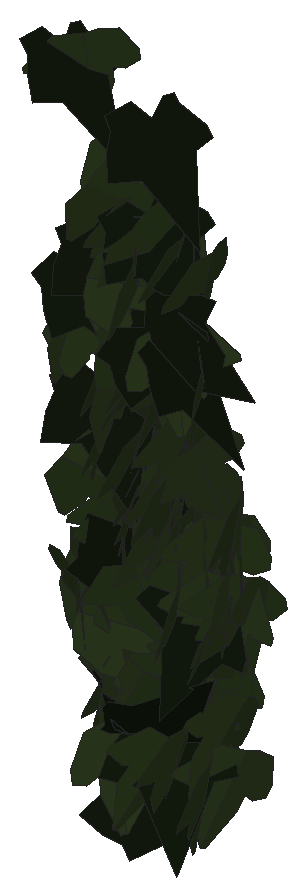
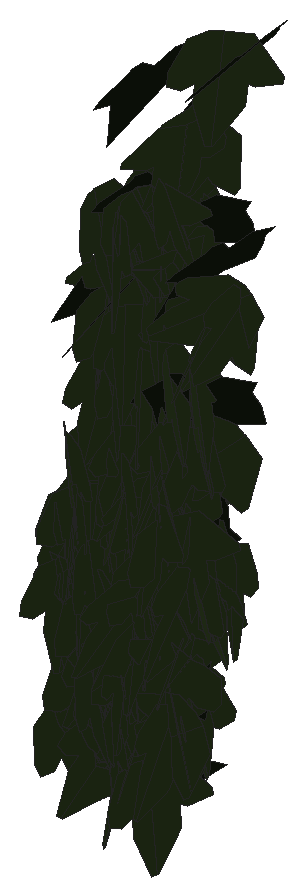
# SketchUp Ruby script. Lengths in inches.
U = 1.inch
M = Sketchup.active_model
def pt(a) = Geom::Point3d.new(a.map { |v| v * U })
def face(e, loops, mat)
  f = e.add_face(loops[0].map { |a| pt(a) })
  loops[1..].each { |l| e.add_face(l.map { |a| pt(a) }).erase! }
  f.material = f.back_material = mat if mat
  f
end
# faces: each face lists its corners as indices into pts; further lists are holes
def faces(e, pts, list, mat = nil) = list.each { |f| face(e, (f[0].is_a?(Array) ? f : [f]).map { |l| l.map { |i| pts[i] } }, mat) }
# xy, xz, yz: faces in a plane at the given z, y or x. An outline is a flat list of corners, or four numbers for a rectangle; further outlines are holes
def ring(l) = l.size == 4 ? [[l[0], l[1]], [l[2], l[1]], [l[2], l[3]], [l[0], l[3]]] : l.each_slice(2).to_a
def flat(e, list, mat, &to3) = list.each { |f| face(e, (f[0].is_a?(Array) ? f : [f]).map { |l| ring(l).map { |u, v| to3.(u, v) } }, mat) }
def xy(e, z, list, mat = nil) = flat(e, list, mat) { |x, y| [x, y, z] }
def xz(e, y, list, mat = nil) = flat(e, list, mat) { |x, z| [x, y, z] }
def yz(e, x, list, mat = nil) = flat(e, list, mat) { |y, z| [x, y, z] }
def lines(e, pts, list) = list.each { |a, b| e.add_line(pt(pts[a]), pt(pts[b])) }
# prism: a flat outline (further loops are holes) pulled along v
def prism(e, loops, v, mat = nil)
  f = face(e, loops, mat); d = Geom::Vector3d.new(v.map { |x| x * U })
  f.pushpull(f.normal.samedirection?(d) ? d.length : -d.length)
end
def box(e, o, s, mat = nil) = prism(e, [[o, [o[0] + s[0], o[1], o[2]], [o[0] + s[0], o[1] + s[1], o[2]], [o[0], o[1] + s[1], o[2]]]], [0, 0, s[2]], mat)
def at(x, y, z, deg = 0) = Geom::Transformation.translation(pt([x, y, z])) * Geom::Transformation.rotation(ORIGIN, Z_AXIS, deg.degrees)
def axes(o, x, y, z) = Geom::Transformation.new([*x, 0, *y, 0, *z, 0, *pt(o).to_a, 1])
def part(name) = M.definitions.add(name)
# library, detail: a bought-in or finely detailed component or shape, given as its bounding box
def library(name, o, s) = part(name).tap { |d| box(d.entities, o, s) }
def detail(e, o, s) = box(e.add_group.entities, o, s)
def put(e, d, t, mat = nil) = e.add_instance(d, t).tap { |i| i.material = mat if mat }
def group(e, t, mat = nil) = e.add_group.tap { |g| g.transformation = t; g.material = mat if mat }.entities
root = M.entities
M.materials.add("efeu1").color = [18, 25, 13]
M.materials.add("efeu2").color = [43, 57, 29]
c1 = part("ivyleaf_10")
p = [[0,0.5,-0.03],[-0.0625,2.02,-0.43],[-0.19,2.01,-0.46],[-0.54,1.05,-0.29],[-0.52,0.625,-0.18],[-0.83,0.76,-0.28],
  [-1.16,0.64,-0.33],[-1.15,0.33,-0.24],[-0.77,-0.39,0.02],[-0.3,-0.51,0.16],[0.04,-0.48,0.23],[-0.02,2.01,-0.4375],
  [-0.06,2.01,-0.43],[0.04,-0.49,0.23],[0.67,-0.49,0.14],[1.38,0.36,-0.2],[1.375,0.51,-0.24],[0.81,0.65,-0.19],
  [0.62,0.59,-0.15],[0.6,1.09,-0.28],[0.5,1.23,-0.31]]
faces(c1.entities,p,[[0,1,2,3,4,5,6,7,8,9,10],[11,12,0,13,14,15,16,17,18,19,20]],"efeu2")
c2 = part("ivyleaf_9")
p = [[1.54,2.16,1.25],[1.36,2.04,1.19],[-0.21,0.99,0.68],[-0.71,1.11,0.82],[-0.85,0.86,0.67],[-0.8,0.17,0.21],
  [-0.9,-0.01,0.1],[-0.67,-0.16,-0.02],[-0.08,-0.08,-0.05],[-0.03,-0.6,-0.4],[0.65,-0.88,-0.66],[0.83,-0.6,-0.49],
  [1.29,-0.42,-0.43],[1.8125,-0.07,-0.26],[1.21,0.44,0.15]]
faces(c2.entities,p,[[0,1,2,3,4,5,6,7,8,9,10,11,12,13,14]],"efeu1")
put(root,c1,axes([15.91,224.3125,216.32],[0.3264,-0.17803,-0.33432],[-0.1434,0.35039,-0.3266],[0.35057,0.30908,0.17768]))
put(root,c1,axes([15.86,224.61,222.82],[-0.35248,-0.35123,-0.049],[0.0485,0.0207,-0.49721],[0.3513,-0.35526,0.01948]))
put(root,c1,axes([15.82,224.41,219.51],[-0.03059,-0.26658,-0.4219],[0.11756,0.40695,-0.26566],[0.48502,-0.11546,0.03778]))
put(root,c1,axes([15.85,225.21,216.42],[-0.05418,-0.35899,-0.34378],[0.08898,0.33323,-0.36199],[0.48903,-0.10041,0.02778]))
put(root,c1,axes([15.89,225.47,214.83],[-0.06009,-0.37722,-0.32264],[0.05139,0.31852,-0.38197],[0.49371,-0.07906,0.00049]))
put(root,c1,axes([15.93,224.9,218.89],[0.17932,-0.454,-0.10828],[-0.01653,0.10974,-0.48753],[0.46644,0.17843,0.02435]))
put(root,c1,axes([15.91,224.83,216.34],[0.21325,-0.44852,0.05793],[0.02073,-0.05429,-0.49661],[0.45177,0.21421,-0.00455]))
put(root,c2,axes([15.6875,224.48,222.81],[0.19731,-0.4431,-0.12137],[0.03083,0.14457,-0.47765],[0.45839,0.18101,0.08437]))
put(root,c1,axes([16.04,225.2,217.02],[-0.27324,-0.41488,0.0567],[-0.01893,-0.0554,-0.49656],[0.41831,-0.2735,0.01457]))
put(root,c1,axes([16.02,224.92,215.07],[0.14589,-0.47813,-0.01052],[0.00012,0.01104,-0.49988],[0.47824,0.14585,0.00334]))
put(root,c1,axes([15.67,224.65,216.34],[0.10547,-0.02634,0.48804],[0.46803,-0.13839,-0.10861],[0.1408,0.47975,-0.00454]))
put(root,c1,axes([15.74,225.4375,214.87],[-0.29243,0.07265,-0.39901],[0.39338,-0.06887,-0.30084],[-0.09867,-0.48988,-0.01688]))
put(root,c1,axes([16.08,225.11,215.03],[0.2408,-0.4293,-0.08783],[-0.033,0.08217,-0.4921],[0.43695,0.24279,0.01124]))
put(root,c1,axes([15.77,225.39,215.61],[0.37606,0.18322,0.27387],[0.25184,0.10818,-0.41818],[-0.2125,0.45247,-0.01092]))
put(root,c1,axes([16.12,225.5,214.13],[-0.20782,-0.45476,-0.00225],[-0.00216,0.00346,-0.49998],[0.45476,-0.20781,-0.0034]))
put(root,c1,axes([15.95,225.38,215.27],[-0.15026,0.18638,0.43896],[0.23977,-0.3683,0.23846],[0.41222,0.28217,0.02131]))
put(root,c1,axes([16.06,225.09,216.44],[-0.45157,-0.11332,-0.18233],[0.18209,0.02273,-0.46511],[0.1137,-0.48646,0.02075]))
put(root,c1,axes([16.15,224.84,217.03],[0.0182,-0.45408,0.20852],[0.06908,-0.20437,-0.45107],[0.49487,0.04522,0.0553]))
put(root,c1,axes([16.2,224.57,218.37],[0.19363,-0.45223,-0.0894],[-0.02976,0.0845,-0.49191],[0.46003,0.19581,0.00581]))
put(root,c1,axes([15.98,224.4,217.82],[-0.2535,-0.15705,-0.40134],[0.34718,0.20147,-0.29812],[0.25535,-0.42982,0.00691]))
put(root,c1,axes([16.24,224.96,218.91],[0.16756,-0.46558,-0.07184],[-0.00818,0.07336,-0.49452],[0.47102,0.1669,0.01696]))
put(root,c2,axes([15.98,224.38,220.26],[0.17839,-0.38394,-0.26602],[0.00861,0.28742,-0.40904],[0.46702,0.14135,0.10916]))
put(root,c1,axes([15.93,224.4,219.62],[-0.15181,-0.18195,-0.44028],[0.42072,0.16558,-0.21349],[0.22349,-0.43529,0.10283]))
put(root,c1,axes([16.24,224.8,216.94],[0.27614,-0.32312,-0.26332],[-0.00852,0.31143,-0.39108],[0.41674,0.22047,0.16649]))
put(root,c1,axes([16.31,225.34,216.55],[-0.18362,-0.46266,0.04723],[-0.01216,-0.04599,-0.49773],[0.4649,-0.18393,0.00563]))
put(root,c1,axes([16.21,224.89,217.96],[-0.18813,-0.38015,-0.26476],[0.11941,0.23631,-0.42415],[0.44761,-0.22281,0.00187]))
put(root,c2,axes([16.09,224.7,218.64],[-0.1689,-0.36114,-0.30175],[0.14601,0.26456,-0.39836],[0.44739,-0.22268,0.01609]))
put(root,c1,axes([16.36,225.32,217.17],[-0.48678,0.07054,0.08983],[-0.09096,-0.00162,-0.49165],[-0.06907,-0.495,0.01441]))
put(root,c1,axes([16.32,224.32,218.91],[0.11409,-0.22495,-0.43172],[0.03363,0.446,-0.2235],[0.48565,0.02196,0.1169]))
put(root,c1,axes([16.4,224.95,217.7],[0.13089,-0.45332,-0.16544],[-0.04834,0.15824,-0.47183],[0.48014,0.13951,-0.0024]))
put(root,c1,axes([16.59,224.62,215.22],[-0.40654,-0.14734,0.25103],[-0.23719,-0.08225,-0.43241],[0.16872,-0.47066,-0.00301]))
put(root,c1,axes([16.47,225.38,215.93],[-0.4607,0.1672,0.09902],[-0.1016,0.00993,-0.48947],[-0.16564,-0.47111,0.02483]))
put(root,c1,axes([16.3,224.71,221.67],[0.20462,0.45615,0.00785],[0.00074,0.00827,-0.49993],[-0.45621,0.2046,0.00271]))
put(root,c1,axes([16.45,225.3125,215.41],[-0.23825,-0.43837,-0.03268],[0.01271,0.03028,-0.49892],[0.4394,-0.23857,-0.00328]))
put(root,c1,axes([16.41,224.8,217.43],[0.23906,-0.439,-0.01132],[-0.00094,0.01238,-0.49985],[0.43915,0.23901,0.0051]))
put(root,c2,axes([16.125,224.86,214.85],[0.34799,-0.35875,0.01413],[0.00766,-0.01226,-0.49979],[0.35895,0.34806,-0.00303]))
put(root,c1,axes([16.4375,224.68,220.97],[0.02425,-0.49125,0.08991],[0.02321,-0.08881,-0.4915],[0.49887,0.02802,0.0185]))
put(root,c1,axes([16.37,224.73,215.57],[-0.03972,-0.34886,-0.35597],[0.12483,0.33876,-0.34592],[0.48253,-0.11635,0.06019]))
put(root,c1,axes([16.46,224.68,218.08],[0.11779,-0.48213,-0.0606],[-0.01222,0.05939,-0.49631],[0.48577,0.1184,0.00221]))
put(root,c1,axes([16.41,225.1,217.53],[-0.2551,0.42938,-0.02363],[0.01258,-0.02001,-0.49944],[-0.42985,-0.25541,-0.0006]))
put(root,c1,axes([16.52,225.25,214.79],[-0.16692,-0.3801,0.27867],[-0.00651,-0.29374,-0.40456],[0.47127,-0.13869,0.09311]))
put(root,c1,axes([16.4,225.51,215.86],[-0.06336,0.47744,-0.1343],[0.00339,-0.13497,-0.48143],[-0.49596,-0.06191,0.01386]))
put(root,c1,axes([16.32,225.57,216.3125],[-0.13509,-0.3874,-0.28578],[0.26213,0.18977,-0.38115],[0.40378,-0.2528,0.15183]))
put(root,c1,axes([16.49,225.38,215.46],[-0.00687,-0.46531,-0.18287],[0.04683,0.18148,-0.46354],[0.49775,-0.0235,0.04109]))
put(root,c1,axes([16.39,224.21,221.44],[-0.20414,-0.27553,-0.36388],[0.19752,0.30603,-0.34254],[0.41148,-0.2836,-0.0161]))
put(root,c1,axes([16.11,225.3,216.16],[0.21621,0.02595,0.45009],[0.43806,0.10591,-0.21653],[-0.10658,0.48796,0.02306]))
put(root,c1,axes([16.53,225.21,216.18],[0.32149,-0.34519,-0.16578],[-0.04518,0.18076,-0.46399],[0.38027,0.31332,0.08503]))
put(root,c1,axes([16.42,224.32,219.85],[0.0741,0.15398,-0.46989],[0.16765,0.43918,0.17035],[0.46519,-0.1828,0.01346]))
put(root,c1,axes([16.28,224.35,216.01],[0.10152,0.12077,0.47446],[0.23427,0.41349,-0.15537],[-0.4299,0.25385,0.02737]))
put(root,c1,axes([16.8,224.47,217.46],[0.20163,-0.07105,0.45199],[-0.42082,0.16508,0.21367],[-0.17959,-0.46658,0.00677]))
put(root,c2,axes([16.35,224.49,220.7],[-0.12105,-0.3658,-0.31864],[0.13884,0.28856,-0.38401],[0.46483,-0.18145,0.03171]))
put(root,c2,axes([16.75,224.8125,213.61],[-0.34451,-0.35475,0.0739],[0.05805,0.04662,0.49443],[-0.35769,0.34925,0.00907]))
put(root,c1,axes([16.61,225.125,214.96],[-0.10935,-0.35626,0.33335],[-0.00065,-0.34152,-0.36519],[0.4879,-0.0803,0.07423]))
put(root,c1,axes([16.45,224.46,214.51],[0.30504,0.39535,0.02547],[0.01524,0.02041,-0.49935],[-0.39588,0.30542,0.00041]))
put(root,c1,axes([16.61,224.98,218.79],[0.13265,-0.40051,-0.26832],[-0.03725,0.26894,-0.41986],[0.48064,0.13138,0.04152]))
put(root,c1,axes([16.67,224.93,220.76],[-0.38481,-0.26177,0.18274],[-0.05538,-0.22714,-0.44198],[0.31441,-0.36039,0.14582]))
put(root,c1,axes([16.65,224.79,220.77],[-0.17812,-0.46386,0.05577],[-0.01443,-0.0542,-0.49684],[0.46698,-0.1786,0.00592]))
put(root,c1,axes([16.58,225.37,214.125],[-0.30917,0.39257,0.01735],[-0.00939,0.01469,-0.4997],[-0.39285,-0.30931,-0.00171]))
put(root,c2,axes([16.45,224.54,216.49],[-0.16588,-0.0569,0.46824],[0.46938,0.02905,0.16982],[-0.04654,0.4959,0.04378]))
put(root,c1,axes([16.76,224.28,220.48],[0.1054,-0.39367,-0.28968],[-0.01924,0.29277,-0.40486],[0.48839,0.09649,0.04657]))
put(root,c1,axes([17,225.4,215.61],[-0.37027,-0.06527,0.3296],[-0.32435,-0.05864,-0.37598],[0.08774,-0.49224,0.00108]))
put(root,c1,axes([16.77,225.11,217.52],[0.29694,-0.35439,-0.19036],[-0.05016,0.20213,-0.45456],[0.39914,0.28905,0.08449]))
put(root,c1,axes([16.44,225.23,214.53],[0.24527,0.20109,0.38653],[0.28437,0.26219,-0.31685],[-0.33012,0.37526,0.01424]))
put(root,c1,axes([16.73,225.43,214.63],[0.36063,-0.33396,-0.09171],[0.00485,0.13727,-0.48076],[0.34629,0.34587,0.10225]))
put(root,c1,axes([16.7,224.79,217.22],[0.00028,0.49208,0.08862],[-0.01815,0.08858,-0.49176],[-0.49967,-0.00294,0.01791]))
put(root,c1,axes([16.75,224.44,216.67],[-0.39705,-0.27846,-0.1217],[0.09958,0.06995,-0.48496],[0.28711,-0.40935,-0.00009]))
put(root,c1,axes([16.63,224.0625,220.43],[0.05117,0.16237,0.47013],[0.07833,0.46408,-0.1688],[-0.49117,0.09092,0.02206]))
put(root,c1,axes([16.83,224.48,219.39],[0.0879,-0.46509,-0.16113],[-0.0233,0.15957,-0.47328],[0.49166,0.09072,0.00638]))
put(root,c1,axes([16.86,224.7,214.47],[-0.07029,-0.39987,0.29183],[-0.02248,-0.29187,-0.40534],[0.49452,-0.07011,0.02306]))
put(root,c1,axes([16.78,224.93,217.73],[-0.16465,-0.37851,-0.28217],[0.11084,0.25949,-0.41277],[0.45892,-0.19848,-0.00154]))
put(root,c1,axes([16.79,224.38,220.9],[-0.14085,-0.39968,-0.26536],[0.10679,0.24351,-0.42344],[0.46771,-0.17596,0.01677]))
put(root,c1,axes([16.875,225.5,215.16],[0.04651,-0.49767,0.01262],[0.00087,-0.01259,-0.49984],[0.49783,0.04652,-0.0003]))
put(root,c1,axes([16.86,225.15,220.47],[0.32952,-0.31532,-0.20491],[-0.02947,0.24996,-0.43203],[0.37489,0.29681,0.14615]))
put(root,c1,axes([17.04,224.88,218.68],[-0.15225,0.30068,0.36934],[-0.30482,0.23641,-0.31811],[-0.36593,-0.32203,0.11132]))
put(root,c1,axes([16.89,224.59,217.16],[-0.0747,-0.46305,-0.17323],[0.03876,0.16917,-0.46891],[0.49287,-0.08348,0.01062]))
put(root,c1,axes([16.78,225.29,214.35],[-0.25924,-0.30767,-0.29688],[0.20494,0.21528,-0.40206],[0.37523,-0.33014,0.01449]))
put(root,c1,axes([16.93,224.9,219.18],[-0.07099,-0.47674,-0.13297],[0.00464,0.13368,-0.48177],[0.49491,-0.06963,-0.01455]))
put(root,c1,axes([16.75,225.11,215.3],[-0.26611,-0.28248,-0.31527],[0.26073,0.18399,-0.38493],[0.33348,-0.36926,0.04938]))
put(root,c1,axes([17,225.39,215.14],[-0.43061,-0.23724,0.09105],[-0.05842,-0.08193,-0.48977],[0.24731,-0.43244,0.04284]))
put(root,c1,axes([16.92,225.47,216.53],[0.04091,-0.4961,-0.04704],[0.00932,0.04795,-0.49761],[0.49824,0.03984,0.01317]))
put(root,c1,axes([16.9375,224.76,217.86],[-0.01238,-0.49279,-0.08369],[0.00786,0.08351,-0.49291],[0.49978,-0.01352,0.00568]))
put(root,c1,axes([16.93,224.8,220.57],[0.13128,-0.48195,-0.02215],[-0.0048,0.02165,-0.49951],[0.48243,0.13137,0.00106]))
put(root,c1,axes([17.03,224.95,215.54],[-0.41958,-0.26059,0.07775],[-0.06265,-0.04649,-0.49388],[0.26463,-0.42418,0.00636]))
put(root,c2,axes([16.71,224.66,220.99],[0.08057,-0.41667,-0.26437],[0.0226,0.27071,-0.41977],[0.49295,0.05569,0.06246]))
put(root,c1,axes([16.99,225.02,217.29],[0.0569,-0.46728,-0.16855],[-0.03442,0.16554,-0.47054],[0.49556,0.06515,-0.01333]))
put(root,c1,axes([16.98,225.31,214.89],[-0.02239,-0.36089,0.34534],[0.00789,-0.3459,-0.36096],[0.49944,-0.01072,0.02118]))
put(root,c1,axes([16.86,225.29,214.85],[-0.43905,0.16072,-0.1772],[0.14785,-0.10887,-0.46507],[-0.18807,-0.46078,0.04807]))
put(root,c1,axes([17.02,225.02,215.49],[0.17858,-0.46487,-0.04481],[-0.01014,0.04411,-0.49795],[0.46691,0.17876,0.00633]))
put(root,c1,axes([17.05,225.32,215.85],[-0.15569,-0.4744,-0.02649],[0.00383,0.02662,-0.49928],[0.47513,-0.15566,-0.00466]))
put(root,c1,axes([16.87,225.38,215.54],[0.38903,-0.26066,0.17525],[0.18451,-0.0361,-0.46331],[0.25418,0.42515,0.0681]))
put(root,c2,axes([16.75,224.48,214.75],[0.42054,0.26834,-0.0337],[0.02778,0.01912,0.49886],[0.26902,-0.42146,0.00117]))
put(root,c2,axes([16.86,224.53,222.27],[0.09848,-0.44445,-0.20679],[-0.01597,0.2079,-0.45445],[0.48995,0.09611,0.02675]))
put(root,c1,axes([16.91,225.15,217.24],[-0.26501,0.32514,-0.27213],[0.15505,-0.22437,-0.41907],[-0.39463,-0.3065,0.0181]))
put(root,c1,axes([17.17,225.1875,215.17],[-0.27002,-0.38097,0.17875],[-0.05934,-0.17579,-0.4643],[0.41661,-0.27196,0.04972]))
put(root,c2,axes([16.96,224.79,214.58],[-0.23113,-0.38581,-0.21847],[0.10857,0.18962,-0.44973],[0.42988,-0.25533,-0.00388]))
put(root,c1,axes([17.04,224.39,217.08],[0.27108,-0.36538,0.20739],[-0.08641,0.19305,0.45306],[-0.41116,-0.28147,0.04152]))
put(root,c1,axes([17.11,224.63,214.64],[0.09276,-0.48879,0.0498],[0.01677,-0.0475,-0.49746],[0.49103,0.09396,0.00758]))
put(root,c1,axes([17.17,225.25,217.05],[-0.38915,-0.313,0.0243],[-0.00531,-0.03213,-0.49894],[0.3139,-0.38858,0.02168]))
put(root,c1,axes([17.16,224.68,218.54],[-0.03899,-0.49834,0.01163],[-0.00161,-0.01154,-0.49986],[0.49847,-0.03902,-0.00071]))
put(root,c1,axes([17.17,224.37,217.97],[0.0599,-0.45693,-0.19397],[-0.01977,0.19303,-0.46082],[0.496,0.06288,0.00506]))
put(root,c1,axes([17.18,224.48,216.54],[0.21152,-0.41478,-0.18226],[-0.04136,0.18262,-0.46361],[0.45116,0.2112,0.04295]))
put(root,c1,axes([17.25,224.77,219.28],[-0.19813,-0.44142,0.12607],[0.00389,-0.13892,-0.4803],[0.45905,-0.18934,0.05848]))
put(root,c1,axes([17.29,225.3,216.32],[0.26577,-0.35086,-0.2372],[-0.06366,0.24376,-0.43189],[0.41871,0.25976,0.0849]))
put(root,c2,axes([17.03,224.24,219.91],[0.04654,-0.13237,-0.47991],[0.08031,0.47768,-0.12397],[0.49131,-0.06554,0.06573]))
put(root,c1,axes([17.31,225.12,216.99],[-0.36593,-0.33652,0.05333],[0.02887,-0.10861,-0.48721],[0.3395,-0.35349,0.09892]))
put(root,c1,axes([17.3,224.88,220.49],[0.04191,-0.49798,-0.01625],[0.00142,0.01643,-0.49973],[0.49824,0.04184,0.00279]))
put(root,c1,axes([17.34,225.06,217.125],[-0.14353,-0.46544,0.11298],[-0.01154,-0.11455,-0.48656],[0.47882,-0.14228,0.02214]))
put(root,c1,axes([17.34,225.05,216.39],[-0.13251,-0.42808,0.22179],[0.00202,-0.23051,-0.44369],[0.48212,-0.11669,0.06282]))
put(root,c1,axes([17.26,225.37,216.21],[0.49756,-0.03091,-0.03847],[-0.03525,0.05025,-0.49622],[0.03454,0.49651,0.04783]))
put(root,c2,axes([17.22,225.01,216.1875],[-0.14059,-0.44794,0.17201],[-0.02392,-0.17248,-0.4687],[0.47923,-0.14002,0.02707]))
put(root,c1,axes([17.35,224.93,216.05],[0.1704,-0.43908,-0.16784],[-0.03685,0.1655,-0.47037],[0.46862,0.17268,0.02405]))
put(root,c1,axes([17.23,224.43,219.68],[0.31187,0.38794,0.04731],[0.00249,0.05856,-0.49655],[-0.39081,0.30996,0.0346]))
put(root,c1,axes([17.34,225.35,216.13],[-0.27353,-0.41145,-0.07674],[0.06308,0.0501,-0.49347],[0.41377,-0.27964,0.0245]))
put(root,c1,axes([17.43,224.6,219.3],[0.19515,-0.32044,-0.33051],[-0.06437,0.33646,-0.36422],[0.45582,0.1847,0.09006]))
put(root,c1,axes([17.4,224.72,214.28],[0.18209,-0.46318,-0.04799],[0.01367,0.05682,-0.49657],[0.46546,0.17953,0.03336]))
put(root,c2,axes([17.17,224.51,219.54],[0.27947,-0.37953,-0.16689],[-0.04503,0.17229,-0.46721],[0.41215,0.27618,0.06212]))
put(root,c1,axes([17.51,225.16,214.27],[-0.20297,-0.41376,0.19391],[-0.04438,-0.19333,-0.45897],[0.45479,-0.20353,0.04176]))
put(root,c1,axes([17.46,225.16,214.9],[0.0057,-0.4304,0.25441],[0.0065,-0.25434,-0.43043],[0.49993,0.00821,0.0027]))
put(root,c1,axes([17.44,224.59,218.32],[-0.15275,-0.4383,-0.1859],[0.08795,0.16589,-0.4634],[0.4679,-0.17428,0.02642]))
put(root,c1,axes([17.46,225.07,216.61],[0.16624,-0.42158,-0.21127],[0.02552,0.23173,-0.44232],[0.47086,0.13628,0.09857]))
put(root,c1,axes([17.48,224.91,216.04],[-0.02797,-0.42243,-0.26603],[0.04066,0.26364,-0.4229],[0.49756,-0.04529,0.0196]))
put(root,c1,axes([17.53,225.15,216.41],[-0.08613,-0.44642,0.20805],[-0.02067,-0.20775,-0.45433],[0.49209,-0.08686,0.01733]))
put(root,c1,axes([17.48,225.15,217.57],[0.36992,-0.32558,-0.08459],[-0.00198,0.12363,-0.48447],[0.33639,0.35876,0.09018]))
put(root,c1,axes([17.45,225.2,216.94],[0.36298,-0.32582,-0.10993],[0.03889,0.19771,-0.4576],[0.34166,0.32365,0.16888]))
put(root,c1,axes([17.52,225.08,217.46],[0.2024,-0.44992,-0.08128],[-0.00242,0.08783,-0.49222],[0.4572,0.19964,0.03338]))
